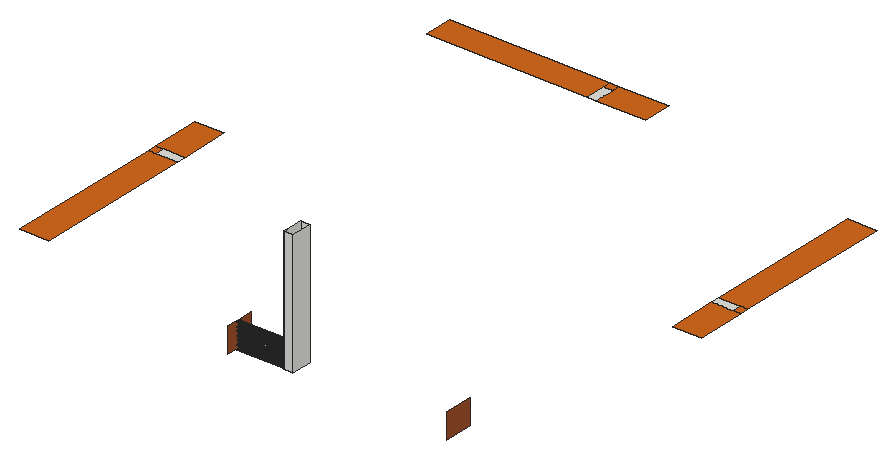
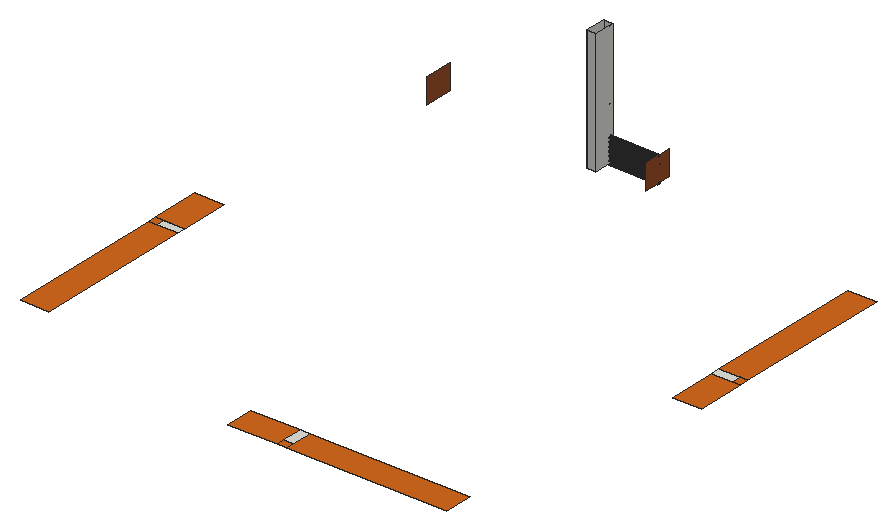
# SketchUp Ruby script. Lengths in inches.
U = 1.inch
M = Sketchup.active_model
def pt(a) = Geom::Point3d.new(a.map { |v| v * U })
def face(e, loops, mat)
  f = e.add_face(loops[0].map { |a| pt(a) })
  loops[1..].each { |l| e.add_face(l.map { |a| pt(a) }).erase! }
  f.material = f.back_material = mat if mat
  f
end
# faces: each face lists its corners as indices into pts; further lists are holes
def faces(e, pts, list, mat = nil) = list.each { |f| face(e, (f[0].is_a?(Array) ? f : [f]).map { |l| l.map { |i| pts[i] } }, mat) }
# xy, xz, yz: faces in a plane at the given z, y or x. An outline is a flat list of corners, or four numbers for a rectangle; further outlines are holes
def ring(l) = l.size == 4 ? [[l[0], l[1]], [l[2], l[1]], [l[2], l[3]], [l[0], l[3]]] : l.each_slice(2).to_a
def flat(e, list, mat, &to3) = list.each { |f| face(e, (f[0].is_a?(Array) ? f : [f]).map { |l| ring(l).map { |u, v| to3.(u, v) } }, mat) }
def xy(e, z, list, mat = nil) = flat(e, list, mat) { |x, y| [x, y, z] }
def xz(e, y, list, mat = nil) = flat(e, list, mat) { |x, z| [x, y, z] }
def yz(e, x, list, mat = nil) = flat(e, list, mat) { |y, z| [x, y, z] }
def lines(e, pts, list) = list.each { |a, b| e.add_line(pt(pts[a]), pt(pts[b])) }
# prism: a flat outline (further loops are holes) pulled along v
def prism(e, loops, v, mat = nil)
  f = face(e, loops, mat); d = Geom::Vector3d.new(v.map { |x| x * U })
  f.pushpull(f.normal.samedirection?(d) ? d.length : -d.length)
end
def box(e, o, s, mat = nil) = prism(e, [[o, [o[0] + s[0], o[1], o[2]], [o[0] + s[0], o[1] + s[1], o[2]], [o[0], o[1] + s[1], o[2]]]], [0, 0, s[2]], mat)
def at(x, y, z, deg = 0) = Geom::Transformation.translation(pt([x, y, z])) * Geom::Transformation.rotation(ORIGIN, Z_AXIS, deg.degrees)
def axes(o, x, y, z) = Geom::Transformation.new([*x, 0, *y, 0, *z, 0, *pt(o).to_a, 1])
def part(name) = M.definitions.add(name)
# library, detail: a bought-in or finely detailed component or shape, given as its bounding box
def library(name, o, s) = part(name).tap { |d| box(d.entities, o, s) }
def detail(e, o, s) = box(e.add_group.entities, o, s)
def put(e, d, t, mat = nil) = e.add_instance(d, t).tap { |i| i.material = mat if mat }
def group(e, t, mat = nil) = e.add_group.tap { |g| g.transformation = t; g.material = mat if mat }.entities
root = M.entities
M.materials.add("[0041_Chocolate]").color = [210, 105, 30]
M.materials.add("[0042_Sienna]").color = [160, 82, 45]
xy(root,706.89,[[72,636.29,132,662.8],[1488,886.83,1548,913.33],[671.48,1452.8125,697.99,1512.8125]])
xy(root,706.89,[[48,169.92,132,636.29],[48,636.29,72,662.8],[48,662.8,132,806.17],[1488,743.45,1572,886.83],[1548,886.83,1572,913.33],
  [1488,913.33,1572,1379.7],[205.11,1452.8125,671.48,1536.8125],[697.99,1452.8125,841.36,1536.8125],[671.48,1512.8125,697.99,1536.8125]],"[0041_Chocolate]")
xz(root,36.8125,[[922.01,706.89,948.52,1066.89]])
xz(root,96.8125,[[922.01,706.89,948.52,1066.89]])
yz(root,778.64,[[12.8125,706.89,44.875,706.89,45.15,707.55,45.73,708.3125,46.5,708.9,47.38,709.27,48.34,709.39,49.29,709.27,50.18,708.9,50.95,708.3125,51.53,707.55,51.8,706.89,96.8125,706.89,96.8125,780,51.19,780,51.53,779.55,51.9,778.66,52.03,777.7,51.9,776.75,51.53,775.86,50.95,775.1,50.18,774.51,49.29,774.14,48.34,774.02,47.38,774.14,46.5,774.51,45.73,775.1,45.15,775.86,44.78,776.75,44.65,777.7,44.78,778.66,45.15,779.55,45.49,780,12.8125,780],[44.875,706.89,51.8,706.89,51.53,707.55,50.95,708.3125,50.18,708.9,49.29,709.27,48.34,709.39,47.38,709.27,46.5,708.9,45.73,708.3125,45.15,707.55],[48.34,774.02,49.29,774.14,50.18,774.51,50.95,775.1,51.53,775.86,51.9,776.75,52.03,777.7,51.9,778.66,51.53,779.55,51.19,780,45.49,780,45.15,779.55,44.78,778.66,44.65,777.7,44.78,776.75,45.15,775.86,45.73,775.1,46.5,774.51,47.38,774.14]],"[0042_Sienna]")
yz(root,922.01,[[[36.8125,706.89,36.8125,1066.89,44.875,1066.89,44.78,1066.66,44.65,1065.7,44.78,1064.75,45.15,1063.86,45.73,1063.1,46.5,1062.51,47.38,1062.14,48.34,1062.02,49.29,1062.14,50.18,1062.51,50.95,1063.1,51.53,1063.86,51.9,1064.75,52.03,1065.7,51.9,1066.66,51.8,1066.89,96.8125,1066.89,96.8125,706.89,51.8,706.89,51.53,707.55,50.95,708.3125,50.18,708.9,49.29,709.27,48.34,709.39,47.38,709.27,46.5,708.9,45.73,708.3125,45.15,707.55,44.875,706.89],[48.34,858.02,49.29,858.14,50.18,858.51,50.95,859.1,51.53,859.86,51.9,860.75,52.03,861.7,51.9,862.66,51.53,863.55,50.95,864.3125,50.18,864.9,49.29,865.27,48.34,865.39,47.38,865.27,46.5,864.9,45.73,864.3125,45.15,863.55,44.78,862.66,44.65,861.7,44.78,860.75,45.15,859.86,45.73,859.1,46.5,858.51,47.38,858.14]],[44.875,706.89,45.15,707.55,45.73,708.3125,46.5,708.9,47.38,709.27,48.34,709.39,49.29,709.27,50.18,708.9,50.95,708.3125,51.53,707.55,51.8,706.89]])
yz(root,948.52,[[36.8125,706.89,96.8125,1066.89]])
yz(root,1414.89,[[12.8125,706.89,96.8125,780]],"[0042_Sienna]")
p = [[922.01,45.15,703.86],[922.01,44.78,704.75],[778.64,44.78,704.75],[778.64,45.15,703.86],[922.01,51.9,704.75],[922.01,51.53,703.86],
  [778.64,51.53,703.86],[778.64,51.9,704.75],[922.01,44.65,705.7],[778.64,44.65,705.7],[922.01,52.03,705.7],[778.64,52.03,705.7],
  [922.01,44.78,706.66],[778.64,44.78,706.66],[922.01,51.9,706.66],[778.64,51.9,706.66],[922.01,44.875,706.89],[922.01,45.15,707.55],
  [778.64,45.15,707.55],[778.64,44.875,706.89],[922.01,51.53,707.55],[922.01,51.8,706.89],[778.64,51.8,706.89],[778.64,51.53,707.55],
  [922.01,45.73,708.3125],[778.64,45.73,708.3125],[922.01,50.95,708.3125],[778.64,50.95,708.3125],[922.01,46.5,708.9],[778.64,46.5,708.9],
  [922.01,50.18,708.9],[778.64,50.18,708.9],[922.01,47.38,709.27],[778.64,47.38,709.27],[922.01,49.29,709.27],[778.64,49.29,709.27],
  [922.01,48.34,709.39],[778.64,48.34,709.39],[922.01,48.34,714.02],[922.01,47.38,714.14],[778.64,47.38,714.14],[778.64,48.34,714.02],
  [922.01,49.29,714.14],[778.64,49.29,714.14],[922.01,46.5,714.51],[778.64,46.5,714.51],[922.01,50.18,714.51],[778.64,50.18,714.51],
  [922.01,45.73,715.1],[778.64,45.73,715.1],[922.01,50.95,715.1],[778.64,50.95,715.1],[922.01,45.15,715.86],[778.64,45.15,715.86],
  [922.01,51.53,715.86],[778.64,51.53,715.86],[922.01,44.78,716.75],[778.64,44.78,716.75],[922.01,51.9,716.75],[778.64,51.9,716.75],
  [922.01,44.65,717.7],[778.64,44.65,717.7],[922.01,52.03,717.7],[778.64,52.03,717.7],[922.01,44.78,718.66],[778.64,44.78,718.66],
  [922.01,51.9,718.66],[778.64,51.9,718.66],[922.01,45.15,719.55],[778.64,45.15,719.55],[922.01,51.53,719.55],[778.64,51.53,719.55],
  [922.01,45.73,720.3125],[778.64,45.73,720.3125],[922.01,50.95,720.3125],[778.64,50.95,720.3125],[922.01,46.5,720.9],[778.64,46.5,720.9],
  [922.01,50.18,720.9],[778.64,50.18,720.9],[922.01,47.38,721.27],[778.64,47.38,721.27],[922.01,49.29,721.27],[778.64,49.29,721.27],
  [922.01,48.34,721.39],[778.64,48.34,721.39],[922.01,48.34,726.02],[922.01,47.38,726.14],[778.64,47.38,726.14],[778.64,48.34,726.02],
  [922.01,49.29,726.14],[778.64,49.29,726.14],[922.01,46.5,726.51],[778.64,46.5,726.51],[922.01,50.18,726.51],[778.64,50.18,726.51],
  [922.01,45.73,727.1],[778.64,45.73,727.1],[922.01,50.95,727.1],[778.64,50.95,727.1],[922.01,45.15,727.86],[778.64,45.15,727.86],
  [922.01,51.53,727.86],[778.64,51.53,727.86],[922.01,44.78,728.75],[778.64,44.78,728.75],[922.01,51.9,728.75],[778.64,51.9,728.75],
  [922.01,44.65,729.7],[778.64,44.65,729.7],[922.01,52.03,729.7],[778.64,52.03,729.7],[922.01,44.78,730.66],[778.64,44.78,730.66],
  [922.01,51.9,730.66],[778.64,51.9,730.66],[922.01,45.15,731.55],[778.64,45.15,731.55],[922.01,51.53,731.55],[778.64,51.53,731.55],
  [922.01,45.73,732.3125],[778.64,45.73,732.3125],[922.01,50.95,732.3125],[778.64,50.95,732.3125],[922.01,46.5,732.9],[778.64,46.5,732.9],
  [922.01,50.18,732.9],[778.64,50.18,732.9],[922.01,47.38,733.27],[778.64,47.38,733.27],[922.01,49.29,733.27],[778.64,49.29,733.27],
  [922.01,48.34,733.39],[778.64,48.34,733.39],[922.01,48.34,738.02],[922.01,47.38,738.14],[778.64,47.38,738.14],[778.64,48.34,738.02],
  [922.01,49.29,738.14],[778.64,49.29,738.14],[922.01,46.5,738.51],[778.64,46.5,738.51],[922.01,50.18,738.51],[778.64,50.18,738.51],
  [922.01,45.73,739.1],[778.64,45.73,739.1],[922.01,50.95,739.1],[778.64,50.95,739.1],[922.01,45.15,739.86],[778.64,45.15,739.86],
  [922.01,51.53,739.86],[778.64,51.53,739.86],[922.01,44.78,740.75],[778.64,44.78,740.75],[922.01,51.9,740.75],[778.64,51.9,740.75],
  [922.01,44.65,741.7],[778.64,44.65,741.7],[922.01,52.03,741.7],[778.64,52.03,741.7],[922.01,44.78,742.66],[778.64,44.78,742.66],
  [922.01,51.9,742.66],[778.64,51.9,742.66],[922.01,45.15,743.55],[778.64,45.15,743.55],[922.01,51.53,743.55],[778.64,51.53,743.55],
  [922.01,45.73,744.3125],[778.64,45.73,744.3125],[922.01,50.95,744.3125],[778.64,50.95,744.3125],[922.01,46.5,744.9],[778.64,46.5,744.9],
  [922.01,50.18,744.9],[778.64,50.18,744.9],[922.01,47.38,745.27],[778.64,47.38,745.27],[922.01,49.29,745.27],[778.64,49.29,745.27],
  [922.01,48.34,745.39],[778.64,48.34,745.39],[922.01,48.34,750.02],[922.01,47.38,750.14],[778.64,47.38,750.14],[778.64,48.34,750.02],
  [922.01,49.29,750.14],[778.64,49.29,750.14],[922.01,46.5,750.51],[778.64,46.5,750.51],[922.01,50.18,750.51],[778.64,50.18,750.51],
  [922.01,45.73,751.1],[778.64,45.73,751.1],[922.01,50.95,751.1],[778.64,50.95,751.1],[922.01,45.15,751.86],[778.64,45.15,751.86],
  [922.01,51.53,751.86],[778.64,51.53,751.86],[922.01,44.78,752.75],[778.64,44.78,752.75],[922.01,51.9,752.75],[778.64,51.9,752.75],
  [922.01,44.65,753.7],[778.64,44.65,753.7],[922.01,52.03,753.7],[778.64,52.03,753.7],[922.01,44.78,754.66],[778.64,44.78,754.66],
  [922.01,51.9,754.66],[778.64,51.9,754.66],[922.01,45.15,755.55],[778.64,45.15,755.55],[922.01,51.53,755.55],[778.64,51.53,755.55],
  [922.01,45.73,756.3125],[778.64,45.73,756.3125],[922.01,50.95,756.3125],[778.64,50.95,756.3125],[922.01,46.5,756.9],[778.64,46.5,756.9],
  [922.01,50.18,756.9],[778.64,50.18,756.9],[922.01,47.38,757.27],[778.64,47.38,757.27],[922.01,49.29,757.27],[778.64,49.29,757.27],
  [922.01,48.34,757.39],[778.64,48.34,757.39],[922.01,48.34,762.02],[922.01,47.38,762.14],[778.64,47.38,762.14],[778.64,48.34,762.02],
  [922.01,49.29,762.14],[778.64,49.29,762.14],[922.01,46.5,762.51],[778.64,46.5,762.51],[922.01,50.18,762.51],[778.64,50.18,762.51],
  [922.01,45.73,763.1],[778.64,45.73,763.1],[922.01,50.95,763.1],[778.64,50.95,763.1],[922.01,45.15,763.86],[778.64,45.15,763.86],
  [922.01,51.53,763.86],[778.64,51.53,763.86],[922.01,44.78,764.75],[778.64,44.78,764.75],[922.01,51.9,764.75],[778.64,51.9,764.75],
  [922.01,44.65,765.7],[778.64,44.65,765.7],[922.01,52.03,765.7],[778.64,52.03,765.7],[922.01,44.78,766.66],[778.64,44.78,766.66],
  [922.01,51.9,766.66],[778.64,51.9,766.66],[922.01,45.15,767.55],[778.64,45.15,767.55],[922.01,51.53,767.55],[778.64,51.53,767.55],
  [922.01,45.73,768.3125],[778.64,45.73,768.3125],[922.01,50.95,768.3125],[778.64,50.95,768.3125],[922.01,46.5,768.9],[778.64,46.5,768.9],
  [922.01,50.18,768.9],[778.64,50.18,768.9],[922.01,47.38,769.27],[778.64,47.38,769.27],[922.01,49.29,769.27],[778.64,49.29,769.27],
  [922.01,48.34,769.39],[778.64,48.34,769.39],[922.01,48.34,774.02],[922.01,47.38,774.14],[778.64,47.38,774.14],[778.64,48.34,774.02],
  [922.01,49.29,774.14],[778.64,49.29,774.14],[922.01,46.5,774.51],[778.64,46.5,774.51],[922.01,50.18,774.51],[778.64,50.18,774.51],
  [922.01,45.73,775.1],[778.64,45.73,775.1],[922.01,50.95,775.1],[778.64,50.95,775.1],[922.01,45.15,775.86],[778.64,45.15,775.86],
  [922.01,51.53,775.86],[778.64,51.53,775.86],[922.01,44.78,776.75],[778.64,44.78,776.75],[922.01,51.9,776.75],[778.64,51.9,776.75],
  [922.01,44.65,777.7],[778.64,44.65,777.7],[922.01,52.03,777.7],[778.64,52.03,777.7],[922.01,44.78,778.66],[778.64,44.78,778.66],
  [922.01,51.9,778.66],[778.64,51.9,778.66],[922.01,45.15,779.55],[778.64,45.15,779.55],[922.01,51.53,779.55],[778.64,51.53,779.55]]
faces(root,p,[[0,1,2,3],[4,5,6,7],[1,8,9,2],[10,4,7,11],[8,12,13,9],[14,10,11,15],[12,16,17,18,19,13],[20,21,14,15,22,23],
  [17,24,25,18],[26,20,23,27],[24,28,29,25],[30,26,27,31],[28,32,33,29],[34,30,31,35],[32,36,37,33],[36,34,35,37],
  [38,39,40,41],[42,38,41,43],[39,44,45,40],[46,42,43,47],[44,48,49,45],[50,46,47,51],[48,52,53,49],[54,50,51,55],
  [52,56,57,53],[58,54,55,59],[56,60,61,57],[62,58,59,63],[60,64,65,61],[66,62,63,67],[64,68,69,65],[70,66,67,71],
  [68,72,73,69],[74,70,71,75],[72,76,77,73],[78,74,75,79],[76,80,81,77],[82,78,79,83],[80,84,85,81],[84,82,83,85],
  [86,87,88,89],[90,86,89,91],[87,92,93,88],[94,90,91,95],[92,96,97,93],[98,94,95,99],[96,100,101,97],[102,98,99,103],
  [100,104,105,101],[106,102,103,107],[104,108,109,105],[110,106,107,111],[108,112,113,109],[114,110,111,115],[112,116,117,113],[118,114,115,119],
  [116,120,121,117],[122,118,119,123],[120,124,125,121],[126,122,123,127],[124,128,129,125],[130,126,127,131],[128,132,133,129],[132,130,131,133],
  [134,135,136,137],[138,134,137,139],[135,140,141,136],[142,138,139,143],[140,144,145,141],[146,142,143,147],[144,148,149,145],[150,146,147,151],
  [148,152,153,149],[154,150,151,155],[152,156,157,153],[158,154,155,159],[156,160,161,157],[162,158,159,163],[160,164,165,161],[166,162,163,167],
  [164,168,169,165],[170,166,167,171],[168,172,173,169],[174,170,171,175],[172,176,177,173],[178,174,175,179],[176,180,181,177],[180,178,179,181],
  [182,183,184,185],[186,182,185,187],[183,188,189,184],[190,186,187,191],[188,192,193,189],[194,190,191,195],[192,196,197,193],[198,194,195,199],
  [196,200,201,197],[202,198,199,203],[200,204,205,201],[206,202,203,207],[204,208,209,205],[210,206,207,211],[208,212,213,209],[214,210,211,215],
  [212,216,217,213],[218,214,215,219],[216,220,221,217],[222,218,219,223],[220,224,225,221],[226,222,223,227],[224,228,229,225],[228,226,227,229],
  [230,231,232,233],[234,230,233,235],[231,236,237,232],[238,234,235,239],[236,240,241,237],[242,238,239,243],[240,244,245,241],[246,242,243,247],
  [244,248,249,245],[250,246,247,251],[248,252,253,249],[254,250,251,255],[252,256,257,253],[258,254,255,259],[256,260,261,257],[262,258,259,263],
  [260,264,265,261],[266,262,263,267],[264,268,269,265],[270,266,267,271],[268,272,273,269],[274,270,271,275],[272,276,277,273],[276,274,275,277],
  [278,279,280,281],[282,278,281,283],[279,284,285,280],[286,282,283,287],[284,288,289,285],[290,286,287,291],[288,292,293,289],[294,290,291,295],
  [292,296,297,293],[298,294,295,299],[296,300,301,297],[302,298,299,303],[300,304,305,301],[306,302,303,307],[304,308,309,305],[310,306,307,311]])
